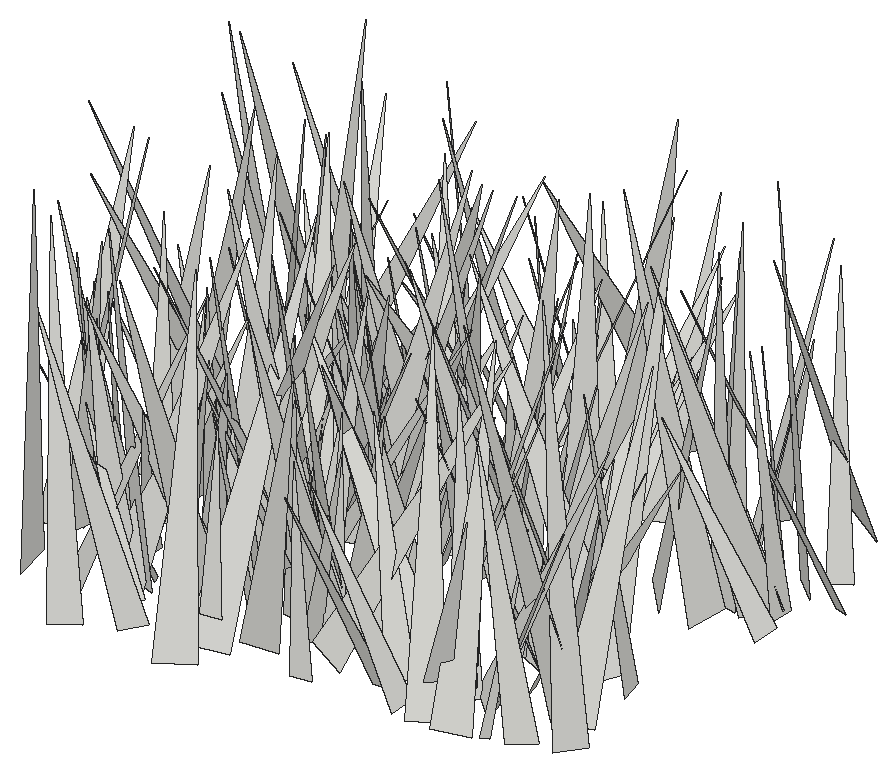
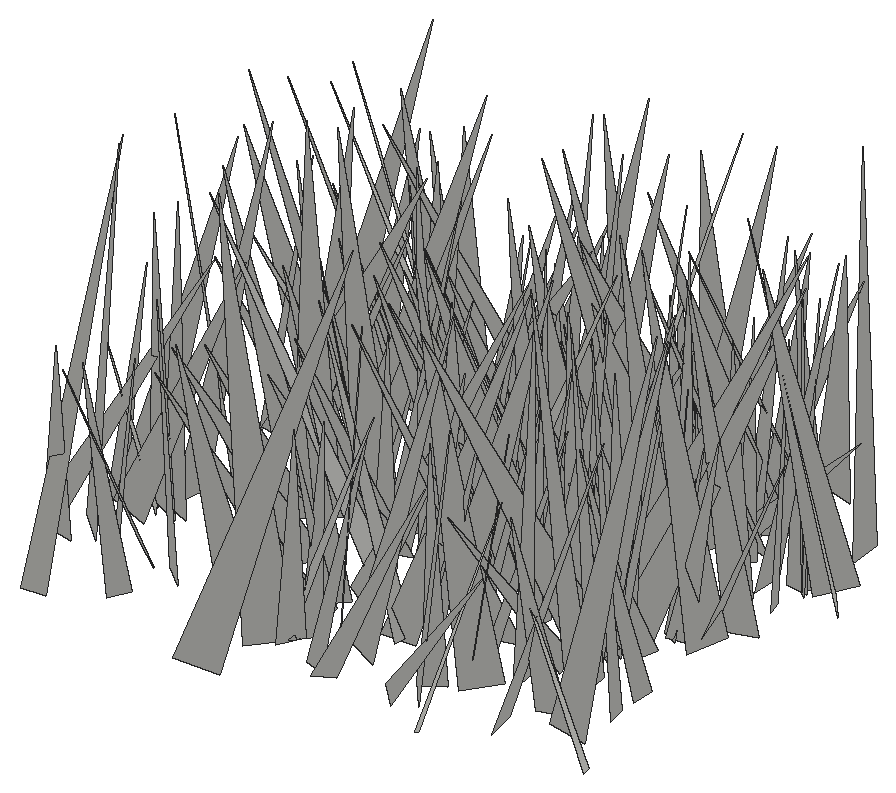
# SketchUp Ruby script. Lengths in inches.
U = 1.inch
M = Sketchup.active_model
def pt(a) = Geom::Point3d.new(a.map { |v| v * U })
def face(e, loops, mat)
  f = e.add_face(loops[0].map { |a| pt(a) })
  loops[1..].each { |l| e.add_face(l.map { |a| pt(a) }).erase! }
  f.material = f.back_material = mat if mat
  f
end
# faces: each face lists its corners as indices into pts; further lists are holes
def faces(e, pts, list, mat = nil) = list.each { |f| face(e, (f[0].is_a?(Array) ? f : [f]).map { |l| l.map { |i| pts[i] } }, mat) }
# xy, xz, yz: faces in a plane at the given z, y or x. An outline is a flat list of corners, or four numbers for a rectangle; further outlines are holes
def ring(l) = l.size == 4 ? [[l[0], l[1]], [l[2], l[1]], [l[2], l[3]], [l[0], l[3]]] : l.each_slice(2).to_a
def flat(e, list, mat, &to3) = list.each { |f| face(e, (f[0].is_a?(Array) ? f : [f]).map { |l| ring(l).map { |u, v| to3.(u, v) } }, mat) }
def xy(e, z, list, mat = nil) = flat(e, list, mat) { |x, y| [x, y, z] }
def xz(e, y, list, mat = nil) = flat(e, list, mat) { |x, z| [x, y, z] }
def yz(e, x, list, mat = nil) = flat(e, list, mat) { |y, z| [x, y, z] }
def lines(e, pts, list) = list.each { |a, b| e.add_line(pt(pts[a]), pt(pts[b])) }
# prism: a flat outline (further loops are holes) pulled along v
def prism(e, loops, v, mat = nil)
  f = face(e, loops, mat); d = Geom::Vector3d.new(v.map { |x| x * U })
  f.pushpull(f.normal.samedirection?(d) ? d.length : -d.length)
end
def box(e, o, s, mat = nil) = prism(e, [[o, [o[0] + s[0], o[1], o[2]], [o[0] + s[0], o[1] + s[1], o[2]], [o[0], o[1] + s[1], o[2]]]], [0, 0, s[2]], mat)
def at(x, y, z, deg = 0) = Geom::Transformation.translation(pt([x, y, z])) * Geom::Transformation.rotation(ORIGIN, Z_AXIS, deg.degrees)
def axes(o, x, y, z) = Geom::Transformation.new([*x, 0, *y, 0, *z, 0, *pt(o).to_a, 1])
def part(name) = M.definitions.add(name)
# library, detail: a bought-in or finely detailed component or shape, given as its bounding box
def library(name, o, s) = part(name).tap { |d| box(d.entities, o, s) }
def detail(e, o, s) = box(e.add_group.entities, o, s)
def put(e, d, t, mat = nil) = e.add_instance(d, t).tap { |i| i.material = mat if mat }
def group(e, t, mat = nil) = e.add_group.tap { |g| g.transformation = t; g.material = mat if mat }.entities
root = M.entities
c1 = part("fur_instance\#9")
p = [[0.8125,0,1.79],[0.67,-0.02,1.48],[0,-0.11,0],[0,0.11,0]]
faces(c1.entities,p,[[0,1,2,3]])
put(root,c1,axes([98.875,26.16,-27.1],[-4.66477,5.25581,1.41142],[5.28211,4.8201,-0.49149],[1.30953,-0.72026,7.01013]))
put(root,c1,axes([96.17,27.25,-27.1],[-1.67581,5.69721,1.32161],[5.39716,0.9769,2.63242],[-2.25291,-1.89755,5.32325]))
put(root,c1,axes([106.84,28.72,-27.1],[-4.54566,0.43172,0.55069],[0.54174,4.46219,0.97364],[0.44289,-1.02717,4.4611]))
put(root,c1,axes([105.45,29.33,-27.1],[-1.01525,-4.25558,0.24661],[-4.20456,0.95799,-0.77812],[-0.70176,0.41691,4.30525]))
put(root,c1,axes([100.4375,28.84,-27.1],[2.54415,-5.74451,1.38415],[-5.89364,-2.3587,1.04378],[0.42454,1.68081,6.19537]))
put(root,c1,axes([94.2,25.96,-27.1],[-0.66678,7.09806,0.59701],[6.83624,0.46921,2.05647],[-2.00116,-0.76214,6.82627]))
put(root,c1,axes([102.92,28.02,-27.1],[-0.42877,3.87256,1.55947],[4.17346,0.35848,0.25729],[-0.1042,-1.57711,3.88772]))
put(root,c1,axes([90.58,28.6875,-27.1],[7.19679,1.10507,2.93039],[1.40985,-7.70082,-0.55845],[-2.79655,-1.03845,7.25969]))
put(root,c1,axes([107.81,29.17,-27.1],[2.67886,-4.09104,0.57639],[-4.11516,-2.58128,0.80469],[0.36641,0.91951,4.82342]))
put(root,c1,axes([98.91,28.01,-27.1],[-3.06481,2.41196,1.362],[2.48233,3.29293,-0.24563],[1.22908,-0.63618,3.89234]))
put(root,c1,axes([96.72,30.5625,-27.1],[1.44091,-6.85532,1.40735],[-6.89305,-1.6385,-0.92385],[-1.20912,1.1714,6.94393]))
put(root,c1,axes([95.12,28.62,-27.1],[-3.33504,1.53851,0.16438],[1.54705,3.32218,0.29368],[0.02564,-0.33558,3.66104]))
put(root,c1,axes([93.9,29.58,-27.1],[3.52477,-3.78027,2.43443],[-3.94318,-4.08529,-0.63451],[-2.1606,1.28874,5.1295]))
put(root,c1,axes([101.61,31.3,-27.1],[2.47706,-6.70826,1.39737],[-6.69174,-2.68793,-1.04158],[-1.47445,0.92925,7.07472]))
put(root,c1,axes([111.7,29.22,-27.1],[-2.10663,5.00928,1.58804],[5.23429,1.84857,1.1125],[-0.46582,-1.88217,5.31913]))
put(root,c1,axes([96.63,31.38,-27.1],[1.14957,-5.99203,1.40359],[-5.68779,-1.57972,-2.08556],[-2.35023,0.89221,5.73379]))
put(root,c1,axes([92.61,28.49,-27.1],[3.5807,5.01538,0.32607],[5.01642,-3.54168,-0.61141],[0.30977,-0.61982,6.13202]))
put(root,c1,axes([101.18,32.28,-27.1],[-2.08812,-6.42397,1.05341],[-6.15561,2.30841,1.87538],[2.11792,0.37569,6.48927]))
put(root,c1,axes([109.32,28.29,-27.1],[-1.91608,6.79372,1.10059],[6.8739,1.94553,-0.04218],[0.33984,-1.04766,7.05863]))
put(root,c1,axes([108.16,28.37,-27.1],[-2.69969,6.39263,0.77147],[6.43614,2.65406,0.5304],[-0.19237,-0.91623,6.91901]))
put(root,c1,axes([93.44,31.64,-27.1],[4.01305,-1.4697,0.35123],[-1.33059,-3.90931,-1.15533],[-0.71618,-0.97223,4.11458]))
put(root,c1,axes([94.71,29.7,-27.1],[-3.5063,-5.04513,2.56803],[-5.65565,3.25438,-1.32851],[0.24851,2.88062,5.99854]))
put(root,c1,axes([101.58,30.29,-27.1],[3.83893,-0.81047,1.08867],[-0.8917,-3.9684,0.19003],[-1.0232,0.41758,3.91895]))
put(root,c1,axes([109.6,30.2,-27.1],[4.10602,0.97464,0.35289],[0.9844,-4.11806,-0.08026],[-0.32469,-0.15985,4.21935]))
put(root,c1,axes([112.16,31.2,-27.1],[-1.47229,-7.46087,2.3597],[-7.72207,0.99683,-1.66627],[-1.2659,2.59656,7.41996]))
put(root,c1,axes([99.125,30.24,-27.1],[0.98464,3.25356,1.70885],[3.23357,-1.6077,1.19779],[-1.74639,-1.14237,3.18127]))
put(root,c1,axes([106.38,30.91,-27.1],[5.98331,3.57339,0.75673],[3.63565,-5.68637,-1.89446],[0.35186,-2.00943,6.70672]))
put(root,c1,axes([110.46,28.74,-27.1],[1.53322,3.39,0.04746],[3.12816,-1.43461,1.41479],[-1.30727,0.54307,3.44111]))
put(root,c1,axes([97.125,28.32,-27.1],[-5.33411,1.7362,0.45715],[1.45522,5.02033,-2.08679],[1.05153,1.85957,5.20696]))
put(root,c1,axes([108.97,30.51,-27.1],[3.86219,5.07234,0.99731],[5.04282,-3.42294,-2.11973],[1.1372,-2.04809,6.01264]))
put(root,c1,axes([105.66,30.08,-27.1],[-2.79772,3.91125,0.86225],[4.00509,2.73873,0.57209],[0.02536,-1.03446,4.77471]))
put(root,c1,axes([93.96,29.45,-27.1],[-0.17372,7.00266,1.70424],[6.95108,0.61311,-1.81067],[1.90374,-1.5996,6.76675]))
put(root,c1,axes([94.68,30.4,-27.1],[-3.03964,-3.22245,0.08473],[-2.53096,2.3136,-2.80576],[-1.9964,1.97328,3.42802]))
put(root,c1,axes([90.39,31.49,-27.1],[5.9168,-1.45412,1.7202],[-1.44139,-6.15974,-0.24915],[-1.73089,0.15879,6.08776]))
put(root,c1,axes([94.91,31.61,-27.1],[4.77554,-0.30271,1.03368],[-0.19329,-4.86277,-0.53104],[-1.0596,-0.47722,4.75556]))
put(root,c1,axes([108.18,30.48,-27.1],[2.13883,-4.28297,3.06723],[-5.00629,-2.68295,-0.2554],[-1.63976,2.60467,4.7805]))
put(root,c1,axes([108.15,31,-27.1],[3.13012,3.09581,1.75638],[3.35561,-3.34662,-0.08138],[-1.18695,-1.29717,4.40172]))
put(root,c1,axes([97.67,34.6875,-27.1],[-5.6893,-5.57398,0.54513],[-5.22917,5.56506,2.3282],[2.00554,-1.30211,7.61688]))
put(root,c1,axes([102.64,29.79,-27.1],[1.86343,6.88556,0.79652],[6.51007,-1.45535,-2.64927],[2.37997,-1.41024,6.62304]))
put(root,c1,axes([90.87,32.05,-27.1],[-1.22041,-5.00142,1.71972],[-5.19067,1.47111,0.5948],[1.01418,1.51086,5.11369]))
put(root,c1,axes([102.03,30.97,-27.1],[3.56835,-1.26097,2.05366],[-1.59686,-3.9854,0.32755],[-1.80488,1.03305,3.77039]))
put(root,c1,axes([90.8,31.99,-27.1],[-3.25997,-4.21096,1.97124],[-4.4396,3.53441,0.20814],[1.38129,1.42168,5.3213]))
put(root,c1,axes([99.1,27.67,-27.1],[-6.13074,4.86156,0.06985],[4.48302,5.69573,-2.94734],[1.88206,2.26926,7.24803]))
put(root,c1,axes([100.23,31.79,-27.1],[-2.15609,-3.98258,0.83043],[-3.73233,1.56246,-2.1972],[-1.61872,1.70208,3.96005]))
put(root,c1,axes([93.35,30.89,-27.1],[2.79379,4.96818,0.70977],[4.95175,-2.59669,-1.31495],[0.8165,-1.25148,5.54607]))
put(root,c1,axes([91.86,32.45,-27.1],[-6.39617,-0.72322,1.67284],[-0.5993,6.59982,0.56183],[1.72113,-0.38959,6.41236]))
put(root,c1,axes([107.12,29.94,-27.1],[5.77926,4.78065,0.80242],[4.74367,-5.8345,0.5954],[-0.99801,-0.04845,7.47663]))
put(root,c1,axes([95.08,32.84,-27.1],[3.8804,-2.67072,0.47699],[-2.66948,-3.90717,-0.15997],[-0.48385,0.13783,4.70793]))
put(root,c1,axes([97.56,32.54,-27.1],[-5.57513,-2.9786,1.92177],[-3.03694,5.86084,0.2736],[1.82819,0.65252,6.315]))
put(root,c1,axes([106.45,30.96,-27.1],[-3.37764,5.82202,0.02709],[5.22944,3.02002,2.9728],[-2.55923,-1.51283,6.03878]))
put(root,c1,axes([113.3,29.92,-27.1],[-7.7657,1.30292,0.44128],[1.14319,7.51969,-2.08465],[0.76515,1.98873,7.59328]))
put(root,c1,axes([99.93,31.21,-27.1],[1.9045,4.44389,1.45881],[4.34306,-2.26488,1.22946],[-1.73613,-0.79091,4.67587]))
put(root,c1,axes([103.48,30.99,-27.1],[-2.78361,3.37072,1.19614],[3.02117,3.0272,-1.49988],[1.91443,0.12385,4.10617]))
put(root,c1,axes([94.83,33.39,-27.1],[-1.17903,-5.46423,1.73554],[-5.62366,1.44698,0.7353],[1.11548,1.51937,5.54141]))
put(root,c1,axes([108.22,34.32,-27.1],[-4.1053,-4.23157,0.31859],[-4.21802,4.11764,0.33835],[0.46467,-0.00766,5.88602]))
put(root,c1,axes([90.63,33.56,-27.1],[4.23333,1.58778,2.03705],[2.11026,-4.38143,-0.97034],[-1.48911,-1.69519,4.41595]))
put(root,c1,axes([99.28,33.24,-27.1],[1.07794,-7.21694,3.00432],[-7.53412,-1.768,-1.54384],[-2.08502,2.65746,7.13181]))
put(root,c1,axes([109.78,34.09,-27.1],[4.97063,-0.22915,0.23226],[-0.15729,-4.7897,-1.3593],[-0.28585,-1.34904,4.78665]))
put(root,c1,axes([89.03,32.14,-27.1],[-4.56158,-4.36485,4.54967],[-5.17144,5.80258,0.38189],[3.60662,2.79958,6.30192]))
put(root,c1,axes([100.9375,33.64,-27.1],[2.11868,-4.0714,0.72457],[-4.11944,-2.00647,0.77101],[0.3627,0.99394,4.52445]))
put(root,c1,axes([96.38,32.29,-27.1],[3.6811,-6.05089,2.6185],[-6.53456,-2.94932,2.37094],[0.87715,3.42178,6.67401]))
put(root,c1,axes([95.3,33.68,-27.1],[6.73019,-3.63445,0.24466],[-3.63894,-6.68481,0.79754],[0.16506,0.81773,7.60715]))
put(root,c1,axes([104.01,33.68,-27.1],[-0.12405,-5.8754,2.10648],[-6.00776,-0.4589,-1.63376],[-1.69244,2.05962,5.64504]))
put(root,c1,axes([89.72,31.31,-27.1],[-4.86903,5.31705,1.90275],[5.12727,5.21523,-1.45307],[2.36698,-0.35954,7.06166]))
put(root,c1,axes([100.45,32.02,-27.1],[-4.55508,3.55475,2.05706],[3.40532,4.98624,-1.07596],[2.29598,-0.34303,5.67691]))
put(root,c1,axes([97.7,35.5,-27.1],[-3.32814,-6.39102,1.50803],[-6.07577,3.63841,2.01068],[2.49085,0.3356,6.91945]))
put(root,c1,axes([100.39,36.41,-27.1],[5.08436,-3.96797,0.13679],[-3.71243,-4.83007,-2.12193],[-1.40762,-1.5937,6.0904]))
put(root,c1,axes([107.71,34.64,-27.1],[2.58278,-6.81445,2.81399],[-6.72051,-3.40212,-2.07037],[-3.03151,1.73634,6.98721]))
put(root,c1,axes([112.31,31.31,-27.1],[-4.09876,5.0884,1.14662],[4.86258,4.25523,-1.50159],[1.8873,0.0873,6.359]))
put(root,c1,axes([103.27,33.65,-27.1],[-3.89447,-3.70378,1.65585],[-4.00703,3.87088,-0.766],[0.63525,1.71028,5.3196]))
put(root,c1,axes([97.26,33.47,-27.1],[3.48145,-1.92251,0.90917],[-2.10367,-3.36896,0.93158],[-0.31179,1.26381,3.86636]))
put(root,c1,axes([109.67,32.26,-27.1],[4.18382,1.92252,0.07247],[1.86113,-4.08842,1.01327],[-0.48737,0.89131,4.49152]))
put(root,c1,axes([98.2,33.87,-27.1],[3.88099,1.49769,1.22771],[1.56049,-4.04689,0.00388],[-1.14683,-0.43823,4.15995]))
put(root,c1,axes([103.68,32.97,-27.1],[3.85077,0.95797,1.10657],[0.6489,-3.90916,1.12606],[-1.31192,0.87829,3.80501]))
put(root,c1,axes([112.32,34.45,-27.1],[-5.31437,-1.63311,1.48269],[-1.72892,5.48589,-0.1545],[1.36976,0.58821,5.55749]))
put(root,c1,axes([92.28,33.6,-27.1],[-1.52023,5.3398,1.43684],[5.52962,1.4775,0.35965],[0.03531,-1.48075,5.54032]))
put(root,c1,axes([109.75,35.04,-27.1],[-3.22494,-3.97651,0.65226],[-4.0077,3.07801,-1.05003],[-0.42001,1.16258,5.01102]))
put(root,c1,axes([110.79,32.97,-27.1],[-3.9364,0.91485,1.26316],[0.41585,3.92071,-1.54367],[1.50319,1.31107,3.73488]))
put(root,c1,axes([103.39,37.03,-27.1],[5.19652,-2.78136,0.42044],[-2.54268,-5.02221,-1.79688],[-1.20313,-1.39929,5.61347]))
put(root,c1,axes([92.28,35.53,-27.1],[3.64013,-0.49009,0.65042],[-0.33955,-3.62113,-0.82821],[-0.74023,-0.74902,3.57838]))
put(root,c1,axes([108.43,33.82,-27.1],[2.40948,7.1196,1.80641],[7.28749,-2.07931,-1.52526],[0.91887,-2.17835,7.35989]))
put(root,c1,axes([93.59,35.64,-27.1],[-2.68709,-2.60275,1.28992],[-2.48203,2.97011,0.82256],[1.50922,0.25052,3.6494]))
put(root,c1,axes([95.42,33.73,-27.1],[-1.01475,7.09695,1.79918],[7.31311,1.06925,-0.09303],[0.3496,-1.76734,7.16853]))
put(root,c1,axes([108.11,34.19,-27.1],[-3.37958,0.77927,1.41196],[0.41341,3.58754,-0.99047],[1.55884,0.73803,3.32382]))
put(root,c1,axes([105.96,37.49,-27.1],[-3.1075,-6.9448,0.74353],[-6.98342,3.07514,-0.46373],[-0.12218,0.86773,7.5942]))
put(root,c1,axes([111.23,34.8,-27.1],[-3.57057,6.8988,1.02898],[6.50769,2.8788,3.28081],[-2.51043,-2.34953,7.04122]))
put(root,c1,axes([93.41,37.78,-27.1],[0.03934,-7.1777,0.79174],[-6.87762,-0.27857,-2.18369],[-2.20103,0.74216,6.83757]))
put(root,c1,axes([95,36.7,-27.1],[-3.02685,-7.70536,1.30124],[-7.48247,2.45538,-2.86554],[-2.25353,2.19686,7.76679]))
put(root,c1,axes([90.37,35.69,-27.1],[0.14436,6.2225,2.72909],[6.68972,0.34776,-1.14678],[1.18962,-2.71069,6.11762]))
put(root,c1,axes([97.26,37.8125,-27.1],[1.41766,-6.83451,0.48866],[-6.53171,-1.19719,2.20513],[2.07029,0.90294,6.62252]))
put(root,c1,axes([98.13,35.66,-27.1],[4.83025,3.81866,0.07193],[3.65702,-4.5907,-1.86288],[1.10161,-1.50398,5.86882]))
put(root,c1,axes([91.07,36.82,-27.1],[-3.67924,-0.76157,0.35539],[-0.68587,3.64327,0.70657],[0.48566,-0.62424,3.6902]))
put(root,c1,axes([108.58,35.74,-27.1],[4.05513,-1.76427,0.28786],[-1.75227,-3.78191,1.50543],[0.35366,1.49134,4.15818]))
put(root,c1,axes([100.34,37.18,-27.1],[-4.77204,-4.71706,0.72174],[-4.75307,4.60775,-1.31181],[-0.42413,1.43592,6.58044]))
put(root,c1,axes([97.88,35.54,-27.1],[4.13014,0.16234,0.60229],[0.00137,-4.03539,1.07832],[-0.62379,1.06603,3.99019]))
put(root,c1,axes([103.34,38.1875,-27.1],[-1.39577,-4.42794,0.41329],[-4.44248,1.40819,0.08395],[0.20461,0.36877,4.64196]))
put(root,c1,axes([92.16,37.42,-27.1],[-1.43466,-3.23484,0.82707],[-3.31328,1.49057,0.08262],[0.41278,0.72144,3.53774]))
put(root,c1,axes([101.8,37.1875,-27.1],[3.71055,0.76796,0.33165],[0.80764,-3.68168,-0.51076],[-0.21789,-0.56867,3.7546]))
put(root,c1,axes([97.42,37.58,-27.1],[3.61055,-0.61097,0.20103],[-0.59508,-3.6081,-0.27795],[-0.24409,-0.24103,3.65131]))
put(root,c1,axes([90.76,37.09,-27.1],[7.15421,-1.9799,2.12173],[-2.22149,-7.36827,0.61487],[-1.86728,1.18029,7.39761]))
put(root,c1,axes([99.53,37.89,-27.1],[-3.854,-0.48704,1.31581],[-0.33639,4.05498,0.51565],[1.36213,-0.37663,3.85028]))
put(root,c1,axes([93.33,38.72,-27.1],[3.21105,-3.45107,0.18225],[-3.45172,-3.21492,-0.06213],[-0.16965,0.09106,4.71348]))
put(root,c1,axes([105.21,36.3,-27.1],[4.98467,2.72403,1.68688],[2.57744,-5.26236,0.88159],[-1.90334,0.00786,5.61161]))
put(root,c1,axes([91.77,37.39,-27.1],[1.42744,-3.53628,2.17287],[-3.81125,-2.02664,-0.79456],[-1.64348,1.62839,3.72982]))
put(root,c1,axes([101.43,36.5,-27.1],[5.10289,-1.83511,1.25864],[-2.13691,-4.91957,1.49087],[-0.62081,1.84972,5.21387]))
put(root,c1,axes([92.49,39.28,-27.1],[3.64505,-0.39812,0.27738],[-0.20845,-3.18305,-1.82936],[-0.43816,-1.79764,3.17779]))
put(root,c1,axes([99.2,36.42,-27.1],[-0.29614,5.30233,1.4786],[4.87042,0.94241,-2.40408],[2.56516,-1.17721,4.73528]))
put(root,c1,axes([106.1,37.02,-27.1],[4.26152,0.65659,1.09682],[0.47447,-4.35714,0.76482],[-1.18701,0.6156,4.24343]))
put(root,c1,axes([100.08,40.43,-27.1],[-0.39765,-7.51588,0.89638],[-7.02687,0.7002,2.75371],[2.81337,0.68655,7.00455]))
put(root,c1,axes([96.21,39.44,-27.1],[6.38697,0.74513,2.00431],[1.2691,-6.40204,-1.66407],[-1.72101,-1.95564,6.21124]))
put(root,c1,axes([104.27,37.51,-27.1],[-7.25051,-1.24633,1.39987],[-1.43303,7.2913,-0.93068],[1.20805,1.16894,7.29774]))
put(root,c1,axes([110.76,35.07,-27.1],[0.70826,8.01559,0.32411],[7.89046,-0.75477,1.42384],[-1.44754,-0.19233,7.91985]))
put(root,c1,axes([92.92,39.37,-27.1],[-2.78076,-3.999,1.01738],[-3.97731,2.92434,0.62365],[1.09912,0.46468,4.83071]))
put(root,c1,axes([100.04,35.77,-27.1],[7.02888,1.27959,1.54515],[0.73768,-6.88381,2.34499],[-1.86566,2.099,6.7486]))
put(root,c1,axes([104.03,38.46,-27.1],[-3.12669,6.25889,3.83958],[6.87271,3.96367,-0.86451],[2.58493,-2.9678,6.9428]))
put(root,c1,axes([92.04,38.96,-27.1],[2.63596,-3.80697,0.02165],[-3.40971,-2.34911,2.07299],[1.69332,1.196,4.14053]))
put(root,c1,axes([96.32,36.85,-27.1],[-3.98192,5.65644,1.02142],[5.69703,4.04883,-0.21229],[0.76316,-0.7113,6.91418]))
put(root,c1,axes([106.88,38.4,-27.1],[4.92232,-5.34816,3.43981],[-5.97476,-5.37881,0.1869],[-2.17654,2.67018,7.26616]))
put(root,c1,axes([98.67,36.73,-27.1],[6.0321,-2.57805,3.10449],[-3.62742,-5.91038,2.14001],[-1.76807,3.33038,6.20104]))
put(root,c1,axes([102.83,39.81,-27.1],[3.43508,-2.31671,0.74566],[-2.27877,-3.51457,-0.42176],[-0.85461,0.05948,4.12177]))
put(root,c1,axes([99.67,39.64,-27.1],[0.21483,-6.37799,2.26736],[-6.52313,-0.80094,-1.63496],[-1.80789,2.13204,6.16862]))
put(root,c1,axes([96.33,38.125,-27.1],[-2.8304,4.89567,0.80261],[4.94903,2.72215,0.8485],[-0.34477,-1.11592,5.59096]))
put(root,c1,axes([98.75,39.08,-27.1],[-3.38469,-3.26483,1.22467],[-3.48648,3.19729,-1.11215],[0.05857,1.65326,4.56929]))
put(root,c1,axes([98.46,37.59,-27.1],[6.56769,-0.93589,1.93904],[-1.50422,-6.44796,1.98276],[-1.54048,2.30611,6.3308]))
put(root,c1,axes([113.5,40.4,-27.1],[-4.40105,0.97982,0.44244],[1.06612,4.21791,1.26401],[0.13855,-1.33202,4.328]))
put(root,c1,axes([96.5,39.43,-27.1],[-5.34365,-1.01248,1.41227],[-1.15776,5.47992,-0.452],[1.29585,0.72082,5.4199]))
put(root,c1,axes([108.83,40.18,-27.1],[5.37674,4.78999,2.15375],[5.23773,-5.117,-1.69543],[-0.38579,-2.71372,6.99849]))
put(root,c1,axes([112.45,41.45,-27.1],[3.31279,-6.01066,2.01721],[-5.81791,-3.7865,-1.72802],[-2.51972,0.84034,6.64203]))
put(root,c1,axes([93.4,40.54,-27.1],[-1.73003,-6.76572,2.01517],[-7.01807,1.42401,-1.24409],[-0.76325,2.2419,6.8717]))
put(root,c1,axes([101.33,37.9,-27.1],[-5.19034,4.80556,0.45379],[4.78626,5.21014,-0.43029],[0.62529,0.00866,7.0603]))
put(root,c1,axes([111.18,40.03,-27.1],[-8.03417,0.61584,1.78735],[0.70083,8.21761,0.3188],[1.75577,-0.4621,8.05143]))
put(root,c1,axes([99.37,43.35,-27.1],[4.98513,-4.06782,0.78587],[-3.3159,-4.65458,-3.05875],[-2.48386,-1.95039,5.66063]))
put(root,c1,axes([103.35,39.39,-27.1],[-3.61899,-3.55384,3.43713],[-4.24844,4.41399,0.09065],[2.52873,2.32973,5.07136]))
put(root,c1,axes([102.11,42,-27.1],[-3.14306,-6.22127,0.26286],[-6.12359,3.03481,-1.39417],[-1.12913,0.859,6.8293]))
put(root,c1,axes([94.89,41.7,-27.1],[4.79188,-1.27621,1.00499],[-1.01396,-4.79557,-1.25507],[-1.26909,-0.98723,4.79746]))
put(root,c1,axes([107.52,38.51,-27.1],[-1.55041,4.4226,0.08121],[4.26043,1.51619,-1.23272],[1.18941,0.33394,4.52145]))
put(root,c1,axes([93.67,39.48,-27.1],[1.68916,7.29229,2.94864],[7.0223,-2.75681,2.79508],[-3.5439,-1.98689,6.94394]))
put(root,c1,axes([103.02,38.67,-27.1],[-0.26942,5.43204,0.24352],[5.36362,0.30555,-0.88154],[0.89325,-0.19629,5.36679]))
put(root,c1,axes([96.1875,42.33,-27.1],[-4.24869,-0.73201,1.00331],[-0.4187,4.21079,1.29914],[1.16925,-1.15205,4.11089]))
put(root,c1,axes([92.08,41.62,-27.1],[6.17707,1.48648,1.9777],[1.80034,-6.34915,-0.85095],[-1.69697,-1.32504,6.29616]))
put(root,c1,axes([90.29,41.25,-27.1],[4.64255,0.07182,0.51653],[0.0806,-4.67045,-0.07504],[-0.51523,-0.08349,4.6425]))
put(root,c1,axes([99.95,41.61,-27.1],[-3.61147,3.35043,1.62323],[3.67501,3.56996,0.80783],[0.59541,-1.71259,4.85958]))
put(root,c1,axes([111.03,41.09,-27.1],[1.52535,6.05061,2.3847],[6.37233,-1.8801,0.69429],[-1.30004,-2.1163,6.20117]))
put(root,c1,axes([113.08,41.73,-27.1],[-4.88413,-0.13594,1.40409],[-0.16648,5.08029,-0.08723],[1.4008,0.12978,4.88524]))
put(root,c1,axes([90.17,42.86,-27.1],[6.17791,2.14602,1.95241],[2.61385,-6.11017,-1.55482],[-1.25898,-2.15507,6.35252]))
put(root,c1,axes([96.7,42.53,-27.1],[-3.36264,-2.39418,1.21792],[-2.41208,3.55006,0.31902],[1.18208,0.43333,4.11555]))
put(root,c1,axes([102.39,40.46,-27.1],[7.40183,3.33475,0.3809],[3.31775,-7.40888,0.39208],[-0.5081,0.20159,8.10888]))
put(root,c1,axes([102.61,42.6,-27.1],[1.94389,-4.04886,0.80465],[-4.08173,-1.75236,1.04312],[0.61659,1.16421,4.36851]))
put(root,c1,axes([112.21,42.1,-27.1],[-0.7555,-5.85213,2.53673],[-5.87032,-0.36099,-2.58111],[-2.49433,2.62211,5.30623]))
put(root,c1,axes([111.65,41.3,-27.1],[2.95559,2.2846,0.71516],[2.24296,-3.03986,0.44126],[-0.83663,-0.07885,3.70947]))
put(root,c1,axes([93.08,40.15,-27.1],[6.18283,-3.26103,2.17206],[-3.91127,-5.37775,3.05962],[-0.2327,3.74499,6.28493]))
put(root,c1,axes([95.04,44.15,-27.1],[3.43044,-6.71204,0.2285],[-6.5076,-3.25868,1.97581],[1.6598,1.09595,7.27431]))
put(root,c1,axes([99.24,43.18,-27.1],[6.07626,0.90493,0.17774],[0.92213,-5.94508,-1.25588],[0.01299,-1.26833,6.01354]))
put(root,c1,axes([98.6,42.25,-27.1],[-2.6227,-3.62693,1.52989],[-3.9333,2.34177,-1.19122],[-0.15598,1.93268,4.31442]))
put(root,c1,axes([92.86,41.61,-27.1],[2.51079,7.35519,2.45383],[7.71335,-2.63218,-0.00261],[-0.79014,-2.32314,7.77193]))
put(root,c1,axes([96.17,41.11,-27.1],[1.82211,6.46965,0.85286],[6.26515,-1.48669,-2.10749],[1.8253,-1.35544,6.38239]))
put(root,c1,axes([111.45,41.22,-27.1],[1.52535,6.57132,1.88983],[6.63248,-1.89273,1.22809],[-1.66251,-1.52175,6.63331]))
put(root,c1,axes([94.18,42.95,-27.1],[-6.46976,-1.55499,2.98827],[-1.52534,7.12153,0.40334],[3.00351,0.26714,6.64177]))
put(root,c1,axes([114.45,43.31,-27.1],[-3.99389,-5.07881,0.29207],[-4.86869,3.70838,-2.09153],[-1.47493,1.51142,6.11318]))
put(root,c1,axes([93.76,41.09,-27.1],[3.8069,0.05751,0.20355],[-0.0416,-3.39391,1.73693],[-0.20739,1.73647,3.38805]))
put(root,c1,axes([101.64,43.625,-27.1],[-4.27511,-3.26782,2.05551],[-3.38668,4.64678,0.34365],[1.85313,0.95347,5.37002]))
put(root,c1,axes([90.7,44.87,-27.1],[-1.04582,-7.4675,1.55674],[-7.62212,0.96116,-0.50998],[-0.30029,1.61039,7.52311]))
put(root,c1,axes([105.11,40.91,-27.1],[-2.16647,5.60636,0.16983],[5.26617,2.09582,-2.00715],[1.93067,0.57445,5.66535]))
put(root,c1,axes([112.53,43.76,-27.1],[-4.94486,-5.49387,2.91837],[-6.02867,5.15162,-0.51692],[1.53451,2.53562,7.37341]))
put(root,c1,axes([96.35,45.12,-27.1],[1.68114,-3.92704,0.2758],[-3.91607,-1.63754,0.5539],[0.40264,0.46985,4.23569]))
put(root,c1,axes([99.78,44.86,-27.1],[-2.51805,-6.35566,1.6356],[-6.55451,2.34778,-0.96776],[-0.32873,1.87181,6.76746]))
put(root,c1,axes([101.77,45.1,-27.1],[3.2467,-2.02133,0.75684],[-1.94033,-3.33216,-0.57574],[-0.94537,-0.10279,3.78092]))
put(root,c1,axes([102.22,43.51,-27.1],[3.63401,0.67625,1.41653],[0.37628,-3.84346,0.86953],[-1.5239,0.6636,3.59267]))
put(root,c1,axes([104.33,42.66,-27.1],[-1.05033,5.0969,0.69056],[4.61293,1.24522,-2.17458],[2.27512,-0.17172,4.72788]))
put(root,c1,axes([110.62,44.86,-27.1],[-2.70575,-2.79772,1.42447],[-3.05403,2.78134,-0.3384],[0.7275,1.27058,3.87735]))
put(root,c1,axes([111.27,48.53,-27.1],[-2.73458,-7.67612,0.26637],[-7.34259,2.69559,2.30041],[2.25392,-0.53168,7.81722]))
put(root,c1,axes([108.17,44.6875,-27.1],[3.30572,4.13092,2.03155],[4.38871,-3.58299,0.14433],[-1.38957,-1.489,5.28881]))
put(root,c1,axes([102.8,45,-27.1],[-4.27144,-3.27285,0.83505],[-3.36103,3.98484,-1.57435],[-0.33515,1.75031,5.14569]))
put(root,c1,axes([92.85,45.83,-27.1],[-6.22564,-1.43503,0.72375],[-1.44178,6.26598,0.02194],[0.71021,0.14105,6.38885]))
put(root,c1,axes([103.62,49.14,-27.1],[3.75973,-6.87339,0.18092],[-6.4988,-3.61971,-2.46477],[-2.2454,-1.03249,7.43666]))
put(root,c1,axes([94.85,47.97,-27.1],[-2.93741,-3.09466,0.01129],[-2.71699,2.58635,2.03327],[1.48156,-1.39259,3.75115]))
put(root,c1,axes([100.41,46.67,-27.1],[-1.40933,-4.17013,0.64925],[-4.20295,1.44894,0.18319],[0.38311,0.55526,4.39803]))
put(root,c1,axes([102.68,46.3,-27.1],[5.49312,-5.94068,1.74056],[-6.16398,-5.4638,0.80479],[-0.57141,1.8305,8.05098]))
put(root,c1,axes([105.65,44.33,-27.1],[-4.4871,3.83069,1.41429],[3.5666,4.69982,-1.41404],[1.98841,0.2144,5.72789]))
put(root,c1,axes([91.99,44.08,-27.1],[-1.75814,5.2069,0.13379],[5.20853,1.75836,0.01288],[0.0306,-0.13088,5.4957]))
put(root,c1,axes([88.56,46.51,-27.1],[3.77978,1.93812,0.15141],[1.88384,-3.56988,-1.33157],[0.48001,-1.25124,4.0336]))
put(root,c1,axes([99.75,46.96,-27.1],[-4.14397,2.00475,0.46664],[2.04964,3.92263,1.34951],[-0.1891,-1.41534,4.40117]))
put(root,c1,axes([102.18,45.74,-27.1],[-4.07522,2.66076,1.05763],[2.66001,4.19896,-0.31421],[1.05952,-0.30776,4.85678]))
put(root,c1,axes([108.82,46.875,-27.1],[3.79566,-1.87078,0.73995],[-1.92959,-3.83243,0.2087],[-0.56925,0.51676,4.2265]))
put(root,c1,axes([96.5,45.85,-27.1],[3.70498,4.05955,2.96614],[3.93602,-4.63444,1.42637],[-3.1282,-1.02317,5.30776]))
put(root,c1,axes([113.22,44.78,-27.1],[-0.43332,5.55714,0.38235],[5.39105,0.32188,1.43136],[-1.40165,-0.47995,5.3871]))
put(root,c1,axes([97.22,46.57,-27.1],[-2.6027,-3.00196,0.39616],[-2.70686,2.07255,-2.07851],[-1.35707,1.62343,3.38609]))
put(root,c1,axes([109.84,44.08,-27.1],[2.78013,5.13783,0.11647],[4.85085,-2.66723,1.86951],[-1.69707,0.79284,5.53456]))
